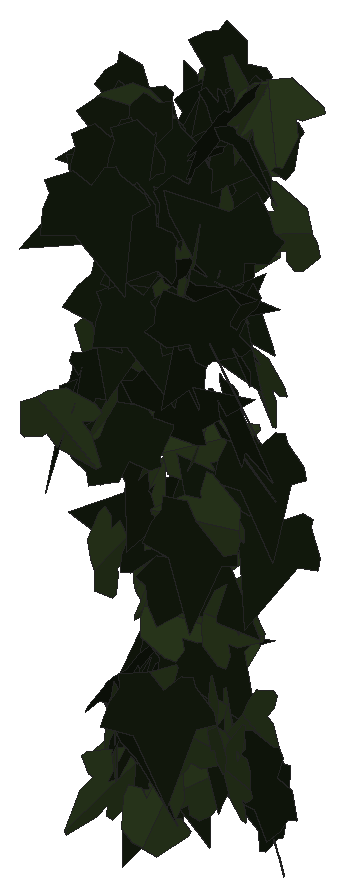
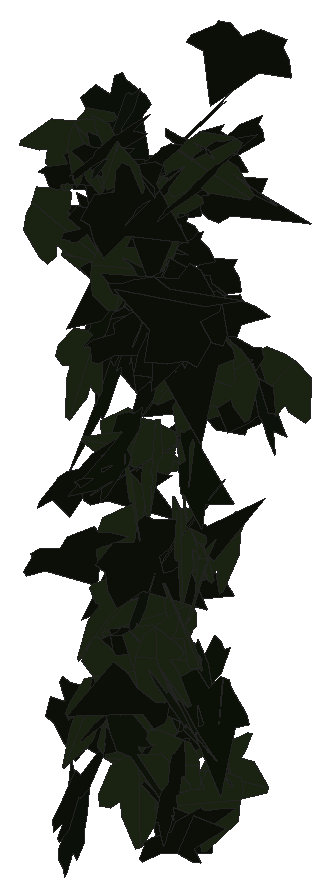
# SketchUp Ruby script. Lengths in inches.
U = 1.inch
M = Sketchup.active_model
def pt(a) = Geom::Point3d.new(a.map { |v| v * U })
def face(e, loops, mat)
  f = e.add_face(loops[0].map { |a| pt(a) })
  loops[1..].each { |l| e.add_face(l.map { |a| pt(a) }).erase! }
  f.material = f.back_material = mat if mat
  f
end
# faces: each face lists its corners as indices into pts; further lists are holes
def faces(e, pts, list, mat = nil) = list.each { |f| face(e, (f[0].is_a?(Array) ? f : [f]).map { |l| l.map { |i| pts[i] } }, mat) }
# xy, xz, yz: faces in a plane at the given z, y or x. An outline is a flat list of corners, or four numbers for a rectangle; further outlines are holes
def ring(l) = l.size == 4 ? [[l[0], l[1]], [l[2], l[1]], [l[2], l[3]], [l[0], l[3]]] : l.each_slice(2).to_a
def flat(e, list, mat, &to3) = list.each { |f| face(e, (f[0].is_a?(Array) ? f : [f]).map { |l| ring(l).map { |u, v| to3.(u, v) } }, mat) }
def xy(e, z, list, mat = nil) = flat(e, list, mat) { |x, y| [x, y, z] }
def xz(e, y, list, mat = nil) = flat(e, list, mat) { |x, z| [x, y, z] }
def yz(e, x, list, mat = nil) = flat(e, list, mat) { |y, z| [x, y, z] }
def lines(e, pts, list) = list.each { |a, b| e.add_line(pt(pts[a]), pt(pts[b])) }
# prism: a flat outline (further loops are holes) pulled along v
def prism(e, loops, v, mat = nil)
  f = face(e, loops, mat); d = Geom::Vector3d.new(v.map { |x| x * U })
  f.pushpull(f.normal.samedirection?(d) ? d.length : -d.length)
end
def box(e, o, s, mat = nil) = prism(e, [[o, [o[0] + s[0], o[1], o[2]], [o[0] + s[0], o[1] + s[1], o[2]], [o[0], o[1] + s[1], o[2]]]], [0, 0, s[2]], mat)
def at(x, y, z, deg = 0) = Geom::Transformation.translation(pt([x, y, z])) * Geom::Transformation.rotation(ORIGIN, Z_AXIS, deg.degrees)
def axes(o, x, y, z) = Geom::Transformation.new([*x, 0, *y, 0, *z, 0, *pt(o).to_a, 1])
def part(name) = M.definitions.add(name)
# library, detail: a bought-in or finely detailed component or shape, given as its bounding box
def library(name, o, s) = part(name).tap { |d| box(d.entities, o, s) }
def detail(e, o, s) = box(e.add_group.entities, o, s)
def put(e, d, t, mat = nil) = e.add_instance(d, t).tap { |i| i.material = mat if mat }
def group(e, t, mat = nil) = e.add_group.tap { |g| g.transformation = t; g.material = mat if mat }.entities
root = M.entities
M.materials.add("efeu1").color = [18, 25, 13]
M.materials.add("efeu2").color = [43, 57, 29]
c1 = part("ivyleaf_9")
p = [[1.54,2.16,1.25],[1.36,2.04,1.19],[-0.21,0.99,0.68],[-0.71,1.11,0.82],[-0.85,0.86,0.67],[-0.8,0.17,0.21],
  [-0.9,-0.01,0.1],[-0.67,-0.16,-0.02],[-0.08,-0.08,-0.05],[-0.03,-0.6,-0.4],[0.65,-0.88,-0.66],[0.83,-0.6,-0.49],
  [1.29,-0.42,-0.43],[1.8125,-0.07,-0.26],[1.21,0.44,0.15]]
faces(c1.entities,p,[[0,1,2,3,4,5,6,7,8,9,10,11,12,13,14]],"efeu1")
c2 = part("ivyleaf_10")
p = [[0,0.5,-0.03],[-0.0625,2.02,-0.43],[-0.19,2.01,-0.46],[-0.54,1.05,-0.29],[-0.52,0.625,-0.18],[-0.83,0.76,-0.28],
  [-1.16,0.64,-0.33],[-1.15,0.33,-0.24],[-0.77,-0.39,0.02],[-0.3,-0.51,0.16],[0.04,-0.48,0.23],[-0.02,2.01,-0.4375],
  [-0.06,2.01,-0.43],[0.04,-0.49,0.23],[0.67,-0.49,0.14],[1.38,0.36,-0.2],[1.375,0.51,-0.24],[0.81,0.65,-0.19],
  [0.62,0.59,-0.15],[0.6,1.09,-0.28],[0.5,1.23,-0.31]]
faces(c2.entities,p,[[0,1,2,3,4,5,6,7,8,9,10],[11,12,0,13,14,15,16,17,18,19,20]],"efeu2")
put(root,c1,axes([33.65,220.62,229.4],[-0.26566,0.06394,-0.41873],[0.38535,-0.16874,-0.27025],[-0.17587,-0.4663,0.04038]))
put(root,c1,axes([33.92,221.37,224.9],[-0.07588,0.49419,0.00447],[-0.00231,0.00417,-0.49998],[-0.4942,-0.0759,0.00165]))
put(root,c2,axes([33.65,221.92,227.08],[-0.23521,0.40176,-0.18238],[0.08168,-0.16346,-0.46541],[-0.43359,-0.24874,0.01126]))
put(root,c1,axes([33.9,222.49,225.56],[-0.44986,0.1522,-0.15641],[0.14146,-0.06952,-0.47451],[-0.16619,-0.47117,0.01949]))
put(root,c1,axes([33.48,222.22,231.24],[0.21353,0.4022,-0.20648],[0.08152,0.19036,0.4551],[0.4447,-0.22802,0.01572]))
put(root,c1,axes([33.76,222.03,228.83],[-0.26528,0.06303,-0.41911],[0.34027,-0.26309,-0.25495],[-0.25267,-0.42049,0.0967]))
put(root,c2,axes([33.85,222.01,227.77],[0.13087,-0.44381,-0.18948],[-0.017,0.19196,-0.46137],[0.48227,0.1272,0.03516]))
put(root,c1,axes([34.2,222.57,231.47],[-0.3035,0.10653,0.3828],[-0.39706,-0.09977,-0.28704],[0.01523,-0.47822,0.14516]))
put(root,c1,axes([33.69,222.09,233.125],[-0.0542,-0.45506,0.19996],[0.02644,-0.2035,-0.45595],[0.49635,-0.03885,0.04613]))
put(root,c1,axes([33.99,221.8,230.61],[0.05613,0.46171,-0.18349],[-0.02331,-0.18201,-0.46511],[-0.49629,0.06077,0.0011]))
put(root,c1,axes([33.89,221.73,231.24],[0.18636,0.45008,0.11269],[0.04978,0.10134,-0.48708],[-0.46129,0.19277,-0.00704]))
put(root,c2,axes([33.65,221.17,229.96],[-0.35748,0.03377,-0.34795],[0.34401,-0.05454,-0.35872],[-0.06218,-0.49587,0.01576]))
put(root,c2,axes([33.67,221.36,223.27],[0.03928,0.0417,-0.49671],[0.32691,0.37397,0.05725],[0.37628,-0.32925,0.00212]))
put(root,c1,axes([34,222.07,225.27],[-0.42508,0.16178,-0.20769],[0.20046,-0.05678,-0.45452],[-0.17065,-0.46968,-0.01659]))
put(root,c2,axes([33.75,220.02,229.33],[-0.41289,-0.08456,-0.26903],[0.26702,0.0362,-0.42118],[0.09071,-0.49147,0.01527]))
put(root,c2,axes([34.09,221.49,233.24],[0.28925,0.18559,-0.36317],[-0.32523,-0.1637,-0.34268],[-0.2461,0.43446,0.02602]))
put(root,c2,axes([33.7,222.07,225.91],[0.39477,-0.2286,-0.20469],[0.17991,-0.09775,0.45616],[-0.24857,-0.4338,0.00508]))
put(root,c1,axes([33.89,222.1875,223.09],[-0.19081,-0.45255,0.09373],[-0.02382,-0.09163,-0.49095],[0.46154,-0.19183,0.01341]))
put(root,c2,axes([33.95,222.59,225.94],[0.01066,-0.18197,0.46559],[0.05374,-0.46258,-0.18202],[0.49699,0.05392,0.0097]))
put(root,c1,axes([34.1,221.71,226.97],[-0.08887,-0.03318,0.49092],[-0.33273,-0.36345,-0.0848],[0.36248,-0.34176,0.04252]))
put(root,c2,axes([34.01,221.11,223.47],[-0.04994,-0.23112,0.44056],[0.00671,-0.44305,-0.23166],[0.49745,-0.01722,0.04736]))
put(root,c2,axes([34.18,222.4375,226.03],[0.3793,-0.10641,-0.30792],[-0.30228,0.0613,-0.39354],[0.1215,0.48469,-0.01783]))
put(root,c2,axes([33.89,221.61,230.45],[-0.2938,-0.2877,-0.28445],[0.23069,0.16966,-0.40988],[0.33236,-0.37208,0.03304]))
put(root,c1,axes([34.39,221.91,222.9],[-0.08152,0.13289,0.47507],[-0.41428,0.24297,-0.13906],[-0.26781,-0.4163,0.0705]))
put(root,c1,axes([34.28,220.82,232.29],[-0.40999,-0.16603,0.23311],[-0.21521,-0.08961,-0.44233],[0.18866,-0.46304,0.00202]))
put(root,c2,axes([33.76,221.29,224.35],[0.19946,-0.2029,0.41116],[0.34799,-0.22495,-0.27982],[0.29853,0.39778,0.05147]))
put(root,c2,axes([33.78,222.06,228.41],[-0.12127,0.07091,0.47986],[0.40702,-0.2542,0.14042],[0.26387,0.42468,0.00393]))
put(root,c1,axes([33.89,222.26,223.88],[-0.03312,0.01158,-0.49877],[0.3979,-0.30093,-0.03341],[-0.30096,-0.39914,0.01072]))
put(root,c2,axes([34.06,220.68,226.91],[0.05401,0.03373,-0.49593],[0.05556,0.49531,0.03974],[0.49396,-0.0594,0.04975]))
put(root,c1,axes([34.25,221.06,223.93],[-0.39276,0.27247,-0.14663],[-0.12423,0.07814,0.47797],[0.28338,0.41189,0.00631]))
put(root,c2,axes([33.89,221.64,227.03],[0.43279,-0.18239,-0.17155],[0.15819,-0.06639,0.46965],[-0.19409,-0.46079,0.00024]))
put(root,c1,axes([33.97,221.85,227.59],[-0.01989,-0.38859,0.31401],[0.00396,-0.31438,-0.38878],[0.49959,-0.01298,0.01559]))
put(root,c1,axes([34.52,221.125,233.04],[-0.41669,0.15477,0.22894],[-0.23452,0.02107,-0.44109],[-0.14619,-0.47497,0.05504]))
put(root,c1,axes([34.24,221.65,230.91],[-0.33601,0.2367,-0.28473],[0.2191,-0.18284,-0.41056],[-0.29848,-0.40068,0.01915]))
put(root,c1,axes([34.14,221.4,233.09],[-0.22559,-0.41392,0.16667],[-0.04968,-0.1623,-0.47031],[0.44344,-0.22875,0.0321]))
put(root,c1,axes([34.16,221.1875,230.71],[-0.28713,-0.39373,-0.11193],[0.06605,0.09037,-0.48731],[0.40397,-0.29463,0.00011]))
put(root,c1,axes([33.85,220.6,229.54],[0.17552,0.0893,-0.45959],[0.22993,0.41111,0.16769],[0.40783,-0.27021,0.10324]))
put(root,c1,axes([34.41,220.73,224.58],[-0.02153,0.24073,0.43771],[-0.05977,0.43372,-0.24148],[-0.49595,-0.06273,0.0101]))
put(root,c2,axes([34.3,221.2,229.42],[0.0849,0.27881,-0.40627],[-0.18783,-0.36282,-0.28824],[-0.45553,0.20157,0.04313]))
put(root,c2,axes([34.42,222.02,228.96],[-0.37298,0.21662,0.25291],[-0.22151,0.12214,-0.43129],[-0.24863,-0.43377,0.00485]))
put(root,c1,axes([34.05,221.91,230.15],[0.2793,-0.39732,-0.11885],[-0.06774,0.09766,-0.48567],[0.40915,0.2874,0.00072]))
put(root,c1,axes([34.4375,222.29,227.41],[-0.04758,0.1972,-0.457],[0.03443,-0.45668,-0.20065],[-0.49654,-0.05056,0.02988]))
put(root,c1,axes([34.17,220.75,233.12],[0.05981,-0.45142,-0.20651],[-0.04029,0.2029,-0.4552],[0.49477,0.07109,-0.0121]))
put(root,c1,axes([34.55,220.61,228.65],[-0.46811,-0.14287,0.10227],[0.0996,0.024,0.48939],[-0.14475,0.47855,0.00599]))
put(root,c1,axes([34.48,222.67,233.05],[-0.06487,0.13269,-0.47769],[0.11282,-0.46517,-0.14453],[-0.48277,-0.12654,0.03042]))
put(root,c2,axes([34.46,222.24,223.81],[-0.31075,-0.3917,0.0012],[-0.00099,-0.00075,-0.5],[0.39171,-0.31075,-0.00031]))
put(root,c1,axes([34.47,222.68,230.87],[-0.26504,-0.39446,0.15542],[-0.09608,-0.12263,-0.47511],[0.41294,-0.28171,-0.0108]))
put(root,c1,axes([34.37,222.21,230.96],[-0.04676,-0.17028,0.46778],[-0.03685,-0.46737,-0.17381],[0.49644,-0.05073,0.03116]))
put(root,c2,axes([34.14,221.75,223.86],[-0.025,-0.03575,-0.49809],[0.4909,0.08973,-0.03107],[0.09161,-0.49058,0.03061]))
put(root,c1,axes([34.4,221.68,230.53],[-0.0507,-0.41734,-0.27066],[0.06362,0.26438,-0.41959],[0.49334,-0.07699,0.02629]))
put(root,c1,axes([34.49,221.47,231.17],[-0.31538,-0.32197,-0.21649],[0.16696,0.13921,-0.45027],[0.35023,-0.35631,0.0197]))
put(root,c2,axes([34.71,221.7,232.45],[-0.30666,-0.3732,0.12915],[-0.07516,-0.10538,-0.48296],[0.3877,-0.31562,0.00853]))
put(root,c1,axes([34.37,222.08,232.72],[0.15998,-0.46838,-0.07091],[-0.01766,0.0689,-0.49492],[0.47339,0.16085,0.0055]))
put(root,c1,axes([34.45,222.25,226.31],[-0.03545,-0.12967,0.48159],[0.03961,-0.48201,-0.12687],[0.49717,0.02916,0.04444]))
put(root,c1,axes([34.9375,221.84,232.89],[-0.4061,0.08687,-0.27846],[-0.27554,0.0424,0.41507],[0.09573,0.49057,0.01344]))
put(root,c1,axes([34.48,221.77,225.19],[0.29317,0.23642,0.32887],[0.21844,0.24959,-0.37415],[-0.34107,0.36306,0.04306]))
put(root,c1,axes([34.76,221.5,232.61],[0.12231,0.47513,-0.09638],[-0.03424,-0.09069,-0.49051],[-0.4836,0.12659,0.01035]))
put(root,c1,axes([34.95,221.65,231.63],[-0.19961,0.41671,0.19108],[-0.10948,0.15905,-0.46121],[-0.44516,-0.22596,0.02775]))
put(root,c1,axes([34.93,221.97,224.37],[-0.32699,0.37822,0.00542],[-0.00722,0.00092,-0.49995],[-0.37819,-0.32703,0.00486]))
put(root,c2,axes([34.73,222.03,228.45],[0.18123,-0.45221,-0.11251],[-0.02809,0.1099,-0.48696],[0.46515,0.18283,0.01443]))
put(root,c1,axes([34.51,221.65,223.93],[0.07715,-0.44736,-0.20955],[-0.02247,0.2087,-0.45381],[0.4935,0.07944,0.0121]))
put(root,c2,axes([34.66,222.6875,231.85],[-0.00561,-0.20279,0.45699],[0.1069,-0.44694,-0.19702],[0.48841,0.09549,0.04837]))
put(root,c2,axes([35,222.23,225.14],[0.19481,0.13081,0.44152],[-0.40441,-0.18067,0.23197],[0.22023,-0.44749,0.03541]))
put(root,c1,axes([34.55,221.16,233.1],[0.0157,-0.47085,-0.16749],[0.03962,0.16821,-0.46918],[0.49818,0.00146,0.0426]))
put(root,c1,axes([34.63,221.83,231.94],[-0.05978,-0.47318,-0.15009],[0.01156,0.1498,-0.47689],[0.49628,-0.06049,-0.00697]))
put(root,c2,axes([35.12,221.89,227.02],[-0.01379,0.01481,-0.49959],[-0.46637,-0.18013,0.00753],[-0.17975,0.46619,0.01878]))
put(root,c1,axes([34.77,222.76,233.59],[-0.17182,-0.37739,0.27938],[-0.0366,-0.28583,-0.40861],[0.46812,-0.16087,0.0706]))
put(root,c2,axes([34.56,221.35,225.97],[0.10788,0.10749,0.47624],[0.28064,0.38545,-0.15057],[-0.39951,0.29979,0.02284]))
put(root,c1,axes([34.52,220.69,224.47],[0.29828,-0.36324,0.17053],[0.10269,-0.13631,-0.46997],[0.38792,0.3154,-0.00671]))
put(root,c1,axes([34.69,220.79,230.9375],[-0.09526,-0.39073,-0.29708],[0.06828,0.28913,-0.40217],[0.48607,-0.11719,-0.00173]))
put(root,c2,axes([35.14,221.37,223.68],[-0.19717,-0.16534,0.4287],[-0.29407,-0.31304,-0.25599],[0.35305,-0.35309,0.0262]))
put(root,c1,axes([34.75,222.09,228.36],[-0.11651,-0.46241,0.15034],[0.09166,-0.17271,-0.46018],[0.47752,-0.07967,0.12501]))
put(root,c2,axes([34.67,222.4,233.53],[0.40478,-0.0841,0.28122],[0.27768,-0.04554,-0.4133],[0.09513,0.49077,0.00983]))
put(root,c1,axes([34.8,221.37,231.55],[-0.14868,-0.41147,-0.24204],[0.07195,0.2313,-0.4374],[0.47193,-0.1649,-0.00957]))
put(root,c2,axes([34.96,220.61,225.1],[-0.1471,0.3875,0.27966],[-0.10059,0.26094,-0.41448],[-0.46717,-0.1782,0.00119]))
put(root,c2,axes([34.98,221.6,232.3125],[-0.03415,0.33414,0.37038],[-0.12221,0.35433,-0.33093],[-0.48363,-0.11314,0.05747]))
put(root,c1,axes([35.09,222.12,228.13],[-0.40619,-0.27932,0.08363],[-0.07135,-0.04384,-0.49294],[0.2827,-0.41238,-0.00425]))
put(root,c2,axes([34.9,220.62,223.21],[0.14278,0.33876,-0.3389],[0.13266,0.31186,0.36762],[0.46045,-0.1949,-0.00082]))
put(root,c1,axes([35.2,220.9,225.21],[-0.15594,0.4712,0.06043],[-0.02143,0.05656,-0.49633],[-0.47458,-0.15738,0.00256]))
put(root,c1,axes([34.78,221.47,226.76],[0.0124,-0.21434,-0.45156],[0.11576,0.44065,-0.20598],[0.48626,-0.09944,0.06055]))
put(root,c1,axes([34.84,221.75,225.49],[-0.0349,-0.29084,-0.40521],[0.06399,0.40023,-0.29278],[0.49466,-0.07229,0.00928]))
put(root,c1,axes([34.74,222.2,228.76],[0.39323,-0.3088,0.00324],[0.00175,-0.00302,-0.49999],[0.30881,0.39323,-0.00129]))
put(root,c2,axes([34.72,221.53,228.45],[0.10465,0.01848,-0.48858],[0.42713,0.23968,0.10055],[0.23792,-0.43842,0.03438]))
put(root,c1,axes([34.87,221.61,232.35],[0.15557,-0.47476,0.02006],[0.00599,-0.01914,-0.4996],[0.47514,0.15569,-0.00027]))
put(root,c1,axes([35.43,222.17,231.95],[-0.39751,-0.11081,0.28232],[-0.27033,-0.08154,-0.41264],[0.13749,-0.4807,0.00491]))
put(root,c1,axes([34.77,220.98,229.24],[0.12247,-0.05117,0.48206],[0.47301,-0.09621,-0.13039],[0.1061,0.48798,0.02484]))
put(root,c1,axes([34.95,221.6875,231.1],[-0.02389,-0.22581,-0.44546],[0.24475,0.38346,-0.20751],[0.43535,-0.22797,0.09222]))
put(root,c1,axes([35.1,221.24,232.53],[0.13189,-0.39291,-0.27969],[-0.09575,0.26285,-0.41441],[0.47269,0.16288,-0.00591]))
put(root,c2,axes([35.25,221.63,226.01],[-0.0239,0.27763,0.41515],[-0.06896,0.40981,-0.27802],[-0.49465,-0.07054,0.0187]))
put(root,c1,axes([35.1,221.27,230.26],[0.10645,-0.16067,-0.46136],[0.3669,-0.28549,0.18408],[-0.32258,-0.37773,0.05712]))
put(root,c1,axes([35.43,222.49,233.1],[-0.363,-0.30979,0.14921],[-0.10553,-0.10612,-0.47708],[0.32725,-0.37785,0.01166]))
put(root,c1,axes([35.15,221.87,224.46],[0.01,-0.48178,0.13336],[0.03116,-0.13253,-0.48111],[0.49893,0.01793,0.02738]))
put(root,c2,axes([34.99,221.6,231.28],[0.03703,0.02513,-0.49799],[0.46576,0.17655,0.04354],[0.17803,-0.46712,-0.01034]))
put(root,c2,axes([35.1,221.1,231.23],[-0.25787,-0.19718,-0.38029],[0.37514,0.11036,-0.3116],[0.20682,-0.44603,0.09102]))
put(root,c1,axes([35.5,221.51,233.66],[-0.20558,0.40078,-0.21705],[0.09163,-0.19691,-0.45037],[-0.44648,-0.22495,0.00752]))
put(root,c2,axes([35.35,222.33,233.47],[0.07563,-0.46297,0.17303],[0.06671,-0.16388,-0.46765],[0.48972,0.09383,0.03698]))
put(root,c1,axes([35.1,221.87,233.48],[0.35784,-0.34917,-0.00533],[-0.00325,0.00431,-0.49997],[0.3492,0.35786,0.00082]))
put(root,c1,axes([35.32,220.18,232.5],[-0.13124,-0.345,0.33727],[-0.00645,-0.34824,-0.35873],[0.48242,-0.09851,0.08696]))
put(root,c1,axes([35.26,218.99,233.57],[-0.19609,-0.28606,-0.36017],[0.19338,0.30397,-0.34671],[0.41732,-0.27527,-0.00858]))
put(root,c2,axes([35.33,220.95,232.01],[0.36577,-0.30265,0.1569],[0.12004,-0.10104,-0.47474],[0.31907,0.38496,-0.00126]))
put(root,c2,axes([35.27,221.61,232.08],[-0.21802,0.12768,-0.43147],[0.17744,-0.4162,-0.21283],[-0.4135,-0.24592,0.13617]))
put(root,c2,axes([35.61,221.52,223.99],[-0.20625,0.3948,-0.22714],[-0.10225,0.20285,0.44542],[0.44385,0.23018,-0.00294]))
put(root,c2,axes([35.83,220.98,227.9],[-0.00182,0.01284,0.49983],[-0.45589,-0.20531,0.00361],[0.20533,-0.45572,0.01245]))
put(root,c1,axes([35.48,222.55,222.92],[-0.08189,0.01536,0.49301],[-0.1678,-0.47082,-0.0132],[0.46383,-0.16762,0.08227]))
put(root,c1,axes([35.32,222.6,222.54],[-0.02263,-0.07857,0.49327],[0.11982,-0.48021,-0.07099],[0.4849,0.11499,0.04056]))
put(root,c1,axes([35.52,222.5625,227.11],[-0.2321,-0.44285,0.00362],[-0.0006,-0.00377,-0.49999],[0.44287,-0.23209,0.00122]))
put(root,c2,axes([35.53,221.88,224.48],[-0.03197,-0.40215,-0.29538],[0.10341,0.28422,-0.39815],[0.48814,-0.08655,0.065]))
put(root,c1,axes([35.48,221.52,229.34],[0.36154,-0.1849,-0.29172],[-0.2563,0.13947,-0.40603],[0.23152,0.44313,0.00607]))
put(root,c1,axes([35.41,222.33,228.27],[0.02924,-0.49386,-0.07244],[-0.01751,0.07151,-0.49455],[0.49884,0.03145,-0.01311]))
put(root,c1,axes([35.36,221.08,231.08],[-0.07728,-0.24609,-0.42833],[0.20604,0.37798,-0.25433],[0.44897,-0.21581,0.04299]))
put(root,c2,axes([35.6,221.95,229.86],[-0.45293,0.21054,-0.02302],[0.02161,-0.00812,-0.49947],[-0.21069,-0.45344,-0.00175]))
put(root,c1,axes([35.3125,221.76,230.52],[0.13445,-0.35678,0.32347],[0.14461,-0.29043,-0.38044],[0.45936,0.19585,0.02509]))
put(root,c2,axes([35.51,222.35,233.51],[0.32915,0.37339,0.04732],[0.02876,0.03773,-0.49774],[-0.37527,0.33039,0.00337]))
put(root,c1,axes([35.52,220.14,225.63],[-0.23868,-0.36877,-0.23883],[0.11586,0.20935,-0.43903],[0.4238,-0.26492,-0.01448]))
put(root,c1,axes([35.51,220.85,227.83],[-0.03275,-0.49823,0.02634],[-0.00141,-0.02631,-0.49931],[0.49892,-0.03278,0.00032]))
put(root,c1,axes([35.28,220.99,231.14],[0.19496,-0.12888,0.44202],[0.42106,-0.1443,-0.22778],[0.18628,0.46105,0.05227]))
put(root,c1,axes([36.05,221.09,231.89],[-0.01888,0.10543,0.48839],[-0.49678,0.04833,-0.02964],[-0.05346,-0.48636,0.10292]))
put(root,c2,axes([35.7,220.49,224.94],[-0.10632,-0.31736,-0.37146],[0.17122,0.33184,-0.33252],[0.45758,-0.19791,0.03812]))
put(root,c1,axes([35.53,220.74,230.65],[-0.1098,-0.1089,0.47548],[0.48713,0.00096,0.11271],[-0.02546,0.488,0.10589]))
put(root,c2,axes([36.09,220.54,225.16],[-0.20247,0.16197,0.42752],[-0.40447,0.15447,-0.25008],[-0.21309,-0.44711,0.06847]))
put(root,c2,axes([36.18,222.14,231.88],[-0.16625,-0.01037,0.47144],[-0.45475,-0.12872,-0.1632],[0.12475,-0.48304,0.03337]))
put(root,c1,axes([35.93,220.96,230.12],[0.27983,0.06842,-0.40868],[-0.41305,0.08531,-0.26854],[0.03298,0.4879,0.10426]))
put(root,c1,axes([35.79,221.125,231.17],[-0.3354,0.27016,0.25401],[0.14493,-0.21976,0.42509],[0.34133,0.35878,0.0691]))
put(root,c1,axes([36.21,221.58,224],[-0.06703,-0.004,-0.49547],[-0.45514,-0.19712,0.06317],[-0.19584,0.45949,0.02278]))
put(root,c2,axes([35.99,221,224.25],[-0.1954,0.26745,0.37455],[-0.21025,0.31009,-0.33111],[-0.4094,-0.2869,-0.00872]))
